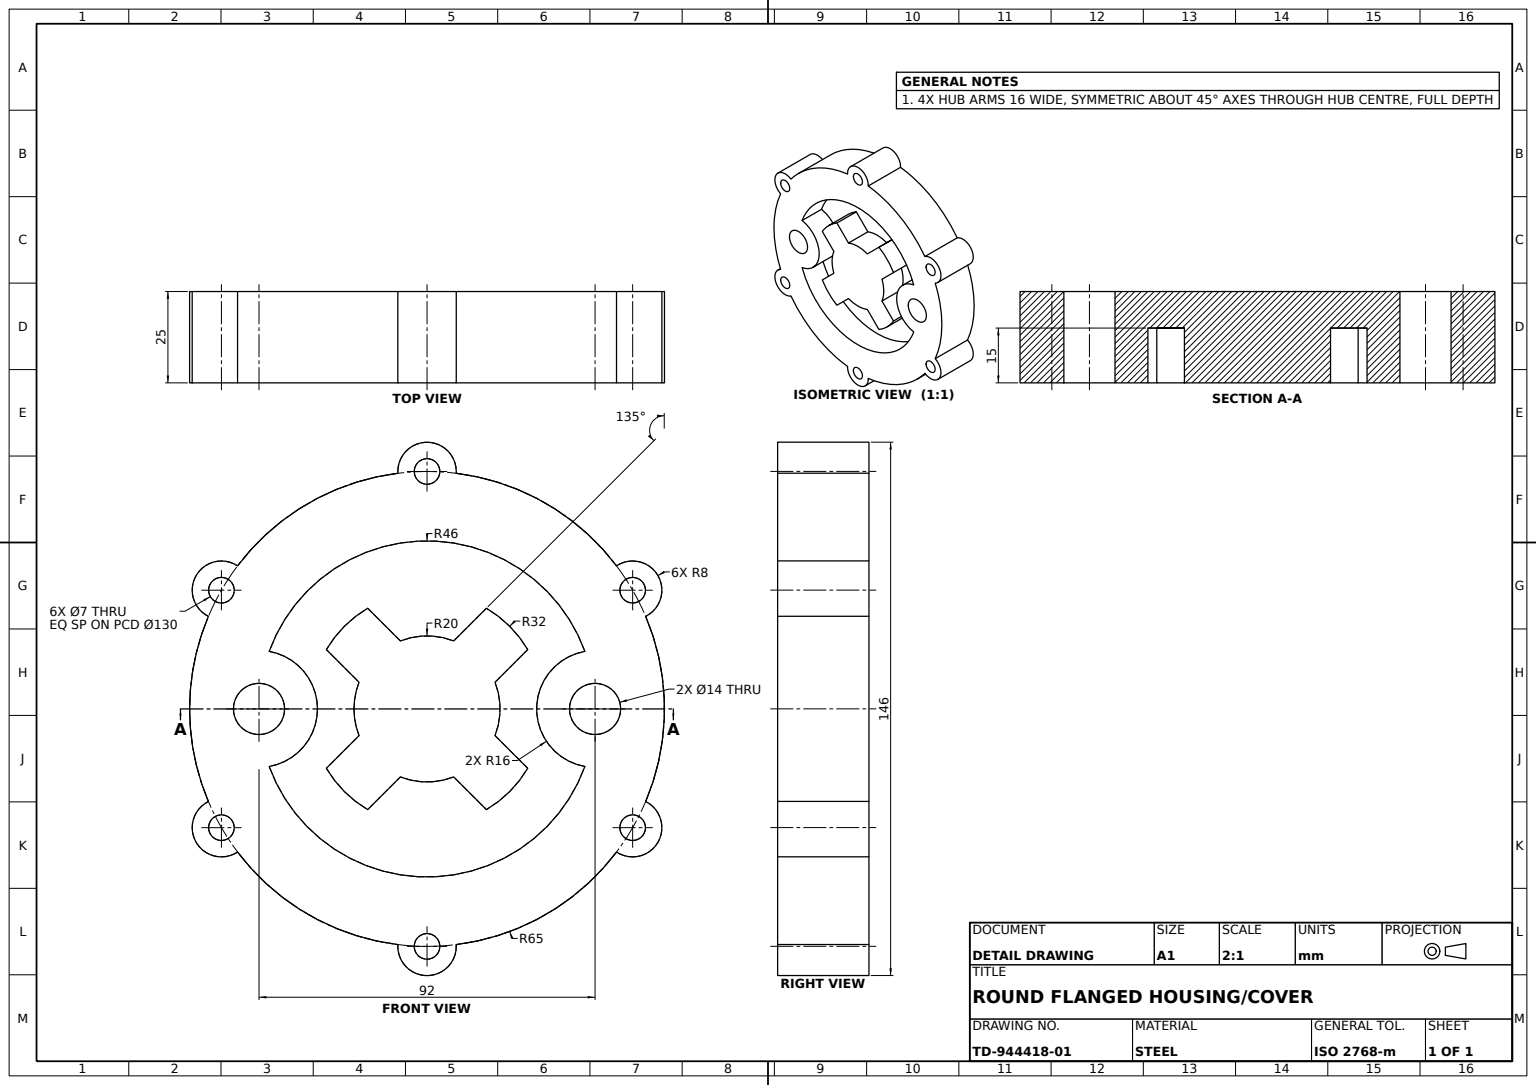
solid
v1 (52.791651,-32.5,25)
v2 (52.791651,-32.5,0)
e1 v1 v2 LINE
v3 (59.791651,-32.5,0)
e2 v3 v2 CIRCLE(AX(P(56.291651,-32.5,0),D(0,0,1),D(1,0,0)),3.5)
v4 (59.791651,-32.5,25)
e3 v4 v3 LINE
e4 v4 v1 CIRCLE(AX(P(56.291651,-32.5,25),D(0,0,1),D(1,0,0)),3.5)
face CYL(AX(P(56.291651,-32.5,25),D(0,0,-1),D(-1,0,0)),3.5) rev [e1 -e2 -e3 e4]
v5 (-16.252048,27.565757,25)
v6 (-16.252048,27.565757,10)
e5 v5 v6 LINE
v7 (-27.565757,16.252048,10)
e6 v6 v7 CIRCLE(AX(P(0,0,10),D(0,0,1),D(1,0,0)),32)
v8 (-27.565757,16.252048,25)
e7 v8 v7 LINE
e8 v5 v8 CIRCLE(AX(P(0,0,25),D(0,0,1),D(1,0,0)),32)
face CYL(AX(P(0,0,25),D(0,0,-1),D(-1,0,0)),32) [e5 e6 -e7 -e8]
v9 (-30,0,10)
v10 (-43.217391,-15.756176,10)
e9 v9 v10 CIRCLE(AX(P(-46,0,10),D(0,0,-1),D(-1,0,0)),16)
v11 (-30,0,25)
e10 v9 v11 LINE
v12 (-43.217391,-15.756176,25)
e11 v11 v12 CIRCLE(AX(P(-46,0,25),D(0,0,-1),D(-1,0,0)),16)
e12 v10 v12 LINE
face CYL(AX(P(-46,0,10),D(0,0,1),D(1,0,0)),16) [-e9 e10 e11 -e12]
v13 (-3.5,-65,25)
v14 (-3.5,-65,0)
e13 v13 v14 LINE
v15 (3.5,-65,25)
e14 v13 v15 CIRCLE(AX(P(0,-65,25),D(0,0,1),D(1,0,0)),3.5)
v16 (3.5,-65,0)
e15 v15 v16 LINE
e16 v14 v16 CIRCLE(AX(P(0,-65,0),D(0,0,1),D(1,0,0)),3.5)
face CYL(AX(P(0,-65,25),D(0,0,-1),D(-1,0,0)),3.5) rev [-e13 e14 e15 -e16]
v17 (-52.791651,32.5,25)
v18 (-52.791651,32.5,0)
e17 v17 v18 LINE
v19 (-59.791651,32.5,0)
e18 v19 v18 CIRCLE(AX(P(-56.291651,32.5,0),D(0,0,1),D(1,0,0)),3.5)
v20 (-59.791651,32.5,25)
e19 v20 v19 LINE
e20 v20 v17 CIRCLE(AX(P(-56.291651,32.5,25),D(0,0,1),D(1,0,0)),3.5)
face CYL(AX(P(-56.291651,32.5,25),D(0,0,-1),D(-1,0,0)),3.5) rev [e17 -e18 -e19 e20]
v21 (8,65,0)
v22 (-8,65,0)
e21 v21 v22 CIRCLE(AX(P(0,65,0),D(0,0,1),D(1,0,0)),8)
v23 (-8,65,25)
e22 v23 v22 LINE
v24 (8,65,25)
e23 v24 v23 CIRCLE(AX(P(0,65,25),D(0,0,1),D(1,0,0)),8)
e24 v24 v21 LINE
face CYL(AX(P(0,65,25),D(0,0,-1),D(-1,0,0)),8) [e21 -e22 -e23 e24]
v25 (7.304627,-18.618336,25)
v26 (7.304627,-18.618336,10)
e25 v25 v26 LINE
v27 (-7.304627,-18.618336,25)
e26 v27 v25 CIRCLE(AX(P(0,0,25),D(0,0,1),D(1,0,0)),20)
v28 (-7.304627,-18.618336,10)
e27 v27 v28 LINE
e28 v28 v26 CIRCLE(AX(P(0,0,10),D(0,0,1),D(1,0,0)),20)
face CYL(AX(P(0,0,25),D(0,0,-1),D(-1,0,0)),20) [-e25 -e26 e27 e28]
v29 (-53,0,0)
v30 (-53,0,25)
e29 v29 v30 LINE
v31 (-39,0,25)
e30 v30 v31 CIRCLE(AX(P(-46,0,25),D(0,0,1),D(-1,0,0)),7)
v32 (-39,0,0)
e31 v32 v31 LINE
e32 v29 v32 CIRCLE(AX(P(-46,0,0),D(0,0,1),D(-1,0,0)),7)
face CYL(AX(P(-46,0,0),D(0,0,1),D(1,0,0)),7) rev [e29 e30 -e31 -e32]
v33 (-59.857719,-25.338774,25)
v34 (-64.291651,-32.5,25)
e33 v33 v34 CIRCLE(AX(P(-56.291651,-32.5,25),D(0,0,1),D(1,0,0)),8)
v35 (-59.857719,-25.338774,0)
e34 v33 v35 LINE
v36 (-64.291651,-32.5,0)
e35 v35 v36 CIRCLE(AX(P(-56.291651,-32.5,0),D(0,0,1),D(1,0,0)),8)
e36 v34 v36 LINE
face CYL(AX(P(-56.291651,-32.5,25),D(0,0,-1),D(-1,0,0)),8) [-e33 e34 e35 -e36]
v37 (59.857719,-25.338774,25)
v38 (59.857719,-25.338774,0)
e37 v37 v38 LINE
v39 (59.857719,25.338774,0)
e38 v38 v39 CIRCLE(AX(P(0,0,0),D(0,0,1),D(1,0,0)),65)
v40 (59.857719,25.338774,25)
e39 v40 v39 LINE
e40 v37 v40 CIRCLE(AX(P(0,0,25),D(0,0,1),D(1,0,0)),65)
face CYL(AX(P(0,0,25),D(0,0,-1),D(-1,0,0)),65) [e37 e38 -e39 -e40]
v41 (7.984838,64.507692,0)
e41 v41 v21 CIRCLE(AX(P(0,65,0),D(0,0,1),D(1,0,0)),8)
v42 (7.984838,64.507692,25)
e42 v42 v24 CIRCLE(AX(P(0,65,25),D(0,0,1),D(1,0,0)),8)
e43 v42 v41 LINE
face CYL(AX(P(0,65,25),D(0,0,-1),D(-1,0,0)),8) [e41 -e24 -e42 e43]
v43 (-51.872881,-39.168918,0)
e44 v36 v43 CIRCLE(AX(P(-56.291651,-32.5,0),D(0,0,1),D(1,0,0)),8)
v44 (-51.872881,-39.168918,25)
e45 v44 v43 LINE
e46 v34 v44 CIRCLE(AX(P(-56.291651,-32.5,25),D(0,0,1),D(1,0,0)),8)
face CYL(AX(P(-56.291651,-32.5,25),D(0,0,-1),D(-1,0,0)),8) [e36 e44 -e45 -e46]
v45 (7.304627,18.618336,25)
v46 (7.304627,18.618336,10)
e47 v45 v46 LINE
v47 (-7.304627,18.618336,10)
e48 v46 v47 CIRCLE(AX(P(0,0,10),D(0,0,1),D(1,0,0)),20)
v48 (-7.304627,18.618336,25)
e49 v48 v47 LINE
e50 v45 v48 CIRCLE(AX(P(0,0,25),D(0,0,1),D(1,0,0)),20)
face CYL(AX(P(0,0,25),D(0,0,-1),D(-1,0,0)),20) [e47 e48 -e49 -e50]
v49 (39,0,0)
v50 (39,0,25)
e51 v49 v50 LINE
v51 (53,0,0)
e52 v51 v49 CIRCLE(AX(P(46,0,0),D(0,0,1),D(1,0,0)),7)
v52 (53,0,25)
e53 v51 v52 LINE
e54 v52 v50 CIRCLE(AX(P(46,0,25),D(0,0,1),D(1,0,0)),7)
face CYL(AX(P(46,0,0),D(0,0,1),D(1,0,0)),7) rev [-e51 -e52 e53 e54]
v53 (-3.5,65,25)
v54 (3.5,65,25)
e55 v53 v54 CIRCLE(AX(P(0,65,25),D(0,0,1),D(1,0,0)),3.5)
e56 v54 v53 CIRCLE(AX(P(0,65,25),D(0,0,1),D(1,0,0)),3.5)
v55 (-52.791651,-32.5,25)
v56 (-59.791651,-32.5,25)
e57 v55 v56 CIRCLE(AX(P(-56.291651,-32.5,25),D(0,0,1),D(1,0,0)),3.5)
e58 v56 v55 CIRCLE(AX(P(-56.291651,-32.5,25),D(0,0,1),D(1,0,0)),3.5)
e59 v15 v13 CIRCLE(AX(P(0,-65,25),D(0,0,1),D(1,0,0)),3.5)
e60 v17 v20 CIRCLE(AX(P(-56.291651,32.5,25),D(0,0,1),D(1,0,0)),3.5)
e61 v31 v30 CIRCLE(AX(P(-46,0,25),D(0,0,1),D(-1,0,0)),7)
v57 (59.791651,32.5,25)
v58 (52.791651,32.5,25)
e62 v57 v58 CIRCLE(AX(P(56.291651,32.5,25),D(0,0,1),D(1,0,0)),3.5)
e63 v58 v57 CIRCLE(AX(P(56.291651,32.5,25),D(0,0,1),D(1,0,0)),3.5)
e64 v50 v52 CIRCLE(AX(P(46,0,25),D(0,0,1),D(1,0,0)),7)
v59 (-43.217391,15.756176,25)
e65 v59 v11 CIRCLE(AX(P(-46,0,25),D(0,0,-1),D(-1,0,0)),16)
v60 (43.217391,15.756176,25)
e66 v60 v59 CIRCLE(AX(P(0,0,25),D(0,0,1),D(1,0,0)),46)
v61 (43.217391,-15.756176,25)
e67 v61 v60 CIRCLE(AX(P(46,0,25),D(0,0,-1),D(1,0,0)),16)
e68 v12 v61 CIRCLE(AX(P(0,0,25),D(0,0,1),D(1,0,0)),46)
v62 (51.872881,39.168918,25)
e69 v62 v42 CIRCLE(AX(P(0,0,25),D(0,0,1),D(1,0,0)),65)
v63 (-7.984838,64.507692,25)
e70 v23 v63 CIRCLE(AX(P(0,65,25),D(0,0,1),D(1,0,0)),8)
v64 (-51.872881,39.168918,25)
e71 v63 v64 CIRCLE(AX(P(0,0,25),D(0,0,1),D(1,0,0)),65)
v65 (-64.291651,32.5,25)
e72 v64 v65 CIRCLE(AX(P(-56.291651,32.5,25),D(0,0,1),D(1,0,0)),8)
v66 (-59.857719,25.338774,25)
e73 v65 v66 CIRCLE(AX(P(-56.291651,32.5,25),D(0,0,1),D(1,0,0)),8)
v67 (-65,0,25)
e74 v66 v67 CIRCLE(AX(P(0,0,25),D(0,0,1),D(1,0,0)),65)
e75 v67 v33 CIRCLE(AX(P(0,0,25),D(0,0,1),D(1,0,0)),65)
v68 (-7.984838,-64.507692,25)
e76 v44 v68 CIRCLE(AX(P(0,0,25),D(0,0,1),D(1,0,0)),65)
v69 (-8,-65,25)
e77 v68 v69 CIRCLE(AX(P(0,-65,25),D(0,0,1),D(1,0,0)),8)
v70 (8,-65,25)
e78 v69 v70 CIRCLE(AX(P(0,-65,25),D(0,0,1),D(1,0,0)),8)
v71 (7.984838,-64.507692,25)
e79 v70 v71 CIRCLE(AX(P(0,-65,25),D(0,0,1),D(1,0,0)),8)
v72 (51.872881,-39.168918,25)
e80 v71 v72 CIRCLE(AX(P(0,0,25),D(0,0,1),D(1,0,0)),65)
e81 v72 v37 CIRCLE(AX(P(56.291651,-32.5,25),D(0,0,1),D(1,0,0)),8)
e82 v40 v62 CIRCLE(AX(P(56.291651,32.5,25),D(0,0,1),D(1,0,0)),8)
e83 v1 v4 CIRCLE(AX(P(56.291651,-32.5,25),D(0,0,1),D(1,0,0)),3.5)
face PLANE(AX(P(28.145826,-16.25,25),D(0,0,1),D(1,0,0))) [-e55 -e56] [-e57 -e58] [-e14 -e59] [-e20 -e60] [-e30 -e61] [-e62 -e63] [-e64 -e54] [-e65 -e66 -e67 -e68 -e11] [e69 e42 e23 e70 e71 e72 e73 e74 e75 e33 e46 e76 e77 e78 e79 e80 e81 e40 e82] [-e83 -e4]
v73 (-8,-65,0)
e84 v69 v73 LINE
v74 (8,-65,0)
e85 v73 v74 CIRCLE(AX(P(0,-65,0),D(0,0,1),D(1,0,0)),8)
e86 v70 v74 LINE
face CYL(AX(P(0,-65,25),D(0,0,-1),D(-1,0,0)),8) [e84 e85 -e86 -e78]
v75 (18.618336,7.304627,25)
v76 (18.618336,7.304627,10)
e87 v75 v76 LINE
v77 (18.618336,-7.304627,25)
e88 v77 v75 CIRCLE(AX(P(0,0,25),D(0,0,1),D(1,0,0)),20)
v78 (18.618336,-7.304627,10)
e89 v77 v78 LINE
e90 v78 v76 CIRCLE(AX(P(0,0,10),D(0,0,1),D(1,0,0)),20)
face CYL(AX(P(0,0,25),D(0,0,-1),D(-1,0,0)),20) [-e87 -e88 e89 e90]
v79 (-27.565757,-16.252048,25)
v80 (-16.252048,-27.565757,25)
e91 v79 v80 CIRCLE(AX(P(0,0,25),D(0,0,1),D(1,0,0)),32)
v81 (-27.565757,-16.252048,10)
e92 v79 v81 LINE
v82 (-16.252048,-27.565757,10)
e93 v81 v82 CIRCLE(AX(P(0,0,10),D(0,0,1),D(1,0,0)),32)
e94 v80 v82 LINE
face CYL(AX(P(0,0,25),D(0,0,-1),D(-1,0,0)),32) [-e91 e92 e93 -e94]
v83 (16.252048,27.565757,25)
v84 (16.252048,27.565757,10)
e95 v83 v84 LINE
e96 v84 v46 LINE
e97 v83 v45 LINE
face PLANE(AX(P(7.304627,18.618336,25),D(0.707106781,-0.707106781,0),D(0.707106781,0.707106781,0))) rev [e95 e96 -e47 -e97]
e98 v80 v27 LINE
e99 v82 v28 LINE
face PLANE(AX(P(-7.304627,-18.618336,25),D(-0.707106781,0.707106781,0),D(-0.707106781,-0.707106781,0))) rev [-e27 -e98 e94 e99]
v85 (51.872881,39.168918,0)
e100 v39 v85 CIRCLE(AX(P(56.291651,32.5,0),D(0,0,1),D(1,0,0)),8)
e101 v62 v85 LINE
face CYL(AX(P(56.291651,32.5,25),D(0,0,-1),D(-1,0,0)),8) [-e82 e39 e100 -e101]
v86 (51.872881,-39.168918,0)
e102 v72 v86 LINE
e103 v86 v38 CIRCLE(AX(P(56.291651,-32.5,0),D(0,0,1),D(1,0,0)),8)
face CYL(AX(P(56.291651,-32.5,25),D(0,0,-1),D(-1,0,0)),8) [e102 e103 -e37 -e81]
v87 (-64.291651,32.5,0)
v88 (-59.857719,25.338774,0)
e104 v87 v88 CIRCLE(AX(P(-56.291651,32.5,0),D(0,0,1),D(1,0,0)),8)
e105 v66 v88 LINE
e106 v65 v87 LINE
face CYL(AX(P(-56.291651,32.5,25),D(0,0,-1),D(-1,0,0)),8) [e104 -e105 -e73 e106]
e107 v85 v41 CIRCLE(AX(P(0,0,0),D(0,0,1),D(1,0,0)),65)
face CYL(AX(P(0,0,25),D(0,0,-1),D(-1,0,0)),65) [e107 -e43 -e69 e101]
v89 (27.565757,16.252048,25)
e108 v75 v89 LINE
e109 v89 v83 CIRCLE(AX(P(0,0,25),D(0,0,1),D(1,0,0)),32)
e110 v48 v5 LINE
v90 (-18.618336,7.304627,25)
e111 v8 v90 LINE
v91 (-20,0,25)
e112 v90 v91 CIRCLE(AX(P(0,0,25),D(0,0,1),D(1,0,0)),20)
v92 (-18.618336,-7.304627,25)
e113 v91 v92 CIRCLE(AX(P(0,0,25),D(0,0,1),D(1,0,0)),20)
e114 v92 v79 LINE
v93 (16.252048,-27.565757,25)
e115 v25 v93 LINE
v94 (27.565757,-16.252048,25)
e116 v93 v94 CIRCLE(AX(P(0,0,25),D(0,0,1),D(1,0,0)),32)
e117 v94 v77 LINE
face PLANE(AX(P(0,0,25),D(0,0,1),D(1,0,0))) [e88 e108 e109 e97 e50 e110 e8 e111 e112 e113 e114 e91 e98 e26 e115 e116 e117]
v95 (-20,0,10)
e118 v91 v95 LINE
v96 (-18.618336,-7.304627,10)
e119 v95 v96 CIRCLE(AX(P(0,0,10),D(0,0,1),D(1,0,0)),20)
e120 v92 v96 LINE
face CYL(AX(P(0,0,25),D(0,0,-1),D(-1,0,0)),20) [e118 e119 -e120 -e113]
v97 (-59.791651,-32.5,0)
e121 v56 v97 LINE
v98 (-52.791651,-32.5,0)
e122 v98 v97 CIRCLE(AX(P(-56.291651,-32.5,0),D(0,0,1),D(1,0,0)),3.5)
e123 v55 v98 LINE
face CYL(AX(P(-56.291651,-32.5,25),D(0,0,-1),D(-1,0,0)),3.5) rev [e121 -e122 -e123 e57]
e124 v32 v29 CIRCLE(AX(P(-46,0,0),D(0,0,1),D(-1,0,0)),7)
face CYL(AX(P(-46,0,0),D(0,0,1),D(1,0,0)),7) rev [-e29 -e124 e31 e61]
v99 (3.5,65,0)
e125 v54 v99 LINE
v100 (-3.5,65,0)
e126 v100 v99 CIRCLE(AX(P(0,65,0),D(0,0,1),D(1,0,0)),3.5)
e127 v53 v100 LINE
face CYL(AX(P(0,65,25),D(0,0,-1),D(-1,0,0)),3.5) rev [e55 e125 -e126 -e127]
v101 (-7.984838,-64.507692,0)
e128 v43 v101 CIRCLE(AX(P(0,0,0),D(0,0,1),D(1,0,0)),65)
e129 v68 v101 LINE
face CYL(AX(P(0,0,25),D(0,0,-1),D(-1,0,0)),65) [e45 e128 -e129 -e76]
v102 (52.791651,32.5,0)
v103 (59.791651,32.5,0)
e130 v102 v103 CIRCLE(AX(P(56.291651,32.5,0),D(0,0,1),D(1,0,0)),3.5)
e131 v58 v102 LINE
e132 v57 v103 LINE
face CYL(AX(P(56.291651,32.5,25),D(0,0,-1),D(-1,0,0)),3.5) rev [-e130 -e131 e63 e132]
v104 (43.217391,15.756176,10)
v105 (-43.217391,15.756176,10)
e133 v104 v105 CIRCLE(AX(P(0,0,10),D(0,0,1),D(1,0,0)),46)
e134 v104 v60 LINE
e135 v105 v59 LINE
face CYL(AX(P(0,0,10),D(0,0,1),D(1,0,0)),46) rev [-e133 e134 e66 -e135]
v106 (-65,0,0)
e136 v67 v106 LINE
e137 v106 v35 CIRCLE(AX(P(0,0,0),D(0,0,1),D(1,0,0)),65)
face CYL(AX(P(0,0,25),D(0,0,-1),D(-1,0,0)),65) [e136 e137 -e34 -e75]
e138 v105 v9 CIRCLE(AX(P(-46,0,10),D(0,0,-1),D(-1,0,0)),16)
face CYL(AX(P(-46,0,10),D(0,0,1),D(1,0,0)),16) [e65 -e10 -e138 e135]
v107 (16.252048,-27.565757,10)
e139 v26 v107 LINE
e140 v93 v107 LINE
face PLANE(AX(P(7.304627,-18.618336,25),D(0.707106781,0.707106781,0),D(-0.707106781,0.707106781,0))) rev [e25 e139 -e140 -e115]
v108 (-51.872881,39.168918,0)
e141 v64 v108 LINE
e142 v108 v87 CIRCLE(AX(P(-56.291651,32.5,0),D(0,0,1),D(1,0,0)),8)
face CYL(AX(P(-56.291651,32.5,25),D(0,0,-1),D(-1,0,0)),8) [-e106 -e72 e141 e142]
v109 (27.565757,-16.252048,10)
e143 v109 v78 LINE
e144 v94 v109 LINE
face PLANE(AX(P(18.618336,-7.304627,25),D(-0.707106781,-0.707106781,0),D(0.707106781,-0.707106781,0))) rev [e143 -e89 -e117 e144]
v110 (-7.984838,64.507692,0)
e145 v22 v110 CIRCLE(AX(P(0,65,0),D(0,0,1),D(1,0,0)),8)
e146 v63 v110 LINE
face CYL(AX(P(0,65,25),D(0,0,-1),D(-1,0,0)),8) [e145 -e146 -e70 e22]
e147 v16 v14 CIRCLE(AX(P(0,-65,0),D(0,0,1),D(1,0,0)),3.5)
face CYL(AX(P(0,-65,25),D(0,0,-1),D(-1,0,0)),3.5) rev [e59 e13 -e147 -e15]
e148 v47 v6 LINE
face PLANE(AX(P(-7.304627,18.618336,25),D(-0.707106781,-0.707106781,0),D(0.707106781,-0.707106781,0))) rev [-e5 -e110 e49 e148]
v111 (7.984838,-64.507692,0)
e149 v74 v111 CIRCLE(AX(P(0,-65,0),D(0,0,1),D(1,0,0)),8)
e150 v71 v111 LINE
face CYL(AX(P(0,-65,25),D(0,0,-1),D(-1,0,0)),8) [-e79 e86 e149 -e150]
e151 v107 v109 CIRCLE(AX(P(0,0,10),D(0,0,1),D(1,0,0)),32)
face CYL(AX(P(0,0,25),D(0,0,-1),D(-1,0,0)),32) [-e144 -e116 e140 e151]
e152 v88 v106 CIRCLE(AX(P(0,0,0),D(0,0,1),D(1,0,0)),65)
face CYL(AX(P(0,0,25),D(0,0,-1),D(-1,0,0)),65) [-e74 e105 e152 -e136]
v112 (-18.618336,7.304627,10)
e153 v90 v112 LINE
e154 v112 v95 CIRCLE(AX(P(0,0,10),D(0,0,1),D(1,0,0)),20)
face CYL(AX(P(0,0,25),D(0,0,-1),D(-1,0,0)),20) [e153 e154 -e118 -e112]
e155 v2 v3 CIRCLE(AX(P(56.291651,-32.5,0),D(0,0,1),D(1,0,0)),3.5)
face CYL(AX(P(56.291651,-32.5,25),D(0,0,-1),D(-1,0,0)),3.5) rev [-e1 e83 e3 -e155]
v113 (27.565757,16.252048,10)
e156 v89 v113 LINE
e157 v113 v84 CIRCLE(AX(P(0,0,10),D(0,0,1),D(1,0,0)),32)
face CYL(AX(P(0,0,25),D(0,0,-1),D(-1,0,0)),32) [-e95 -e109 e156 e157]
e158 v103 v102 CIRCLE(AX(P(56.291651,32.5,0),D(0,0,1),D(1,0,0)),3.5)
e159 v18 v19 CIRCLE(AX(P(-56.291651,32.5,0),D(0,0,1),D(1,0,0)),3.5)
e160 v99 v100 CIRCLE(AX(P(0,65,0),D(0,0,1),D(1,0,0)),3.5)
e161 v97 v98 CIRCLE(AX(P(-56.291651,-32.5,0),D(0,0,1),D(1,0,0)),3.5)
e162 v49 v51 CIRCLE(AX(P(46,0,0),D(0,0,1),D(1,0,0)),7)
e163 v110 v108 CIRCLE(AX(P(0,0,0),D(0,0,1),D(1,0,0)),65)
e164 v111 v86 CIRCLE(AX(P(0,0,0),D(0,0,1),D(1,0,0)),65)
e165 v101 v73 CIRCLE(AX(P(0,-65,0),D(0,0,1),D(1,0,0)),8)
face PLANE(AX(P(28.145826,-16.25,0),D(0,0,1),D(1,0,0))) rev [e158 e130] [e2 e155] [e159 e18] [e160 e126] [e16 e147] [e161 e122] [e162 e52] [-e35 -e137 -e152 -e104 -e142 -e163 -e145 -e21 -e41 -e107 -e100 -e38 -e103 -e164 -e149 -e85 -e165 -e128 -e44] [e32 e124]
face CYL(AX(P(56.291651,32.5,25),D(0,0,-1),D(-1,0,0)),3.5) rev [e131 -e158 -e132 e62]
v114 (43.217391,-15.756176,10)
e166 v10 v114 CIRCLE(AX(P(0,0,10),D(0,0,1),D(1,0,0)),46)
e167 v114 v61 LINE
face CYL(AX(P(0,0,10),D(0,0,1),D(1,0,0)),46) rev [-e166 e12 e68 -e167]
face CYL(AX(P(-56.291651,32.5,25),D(0,0,-1),D(-1,0,0)),3.5) rev [-e17 e60 e19 -e159]
face CYL(AX(P(0,-65,25),D(0,0,-1),D(-1,0,0)),8) [e165 -e84 -e77 e129]
face CYL(AX(P(46,0,0),D(0,0,1),D(1,0,0)),7) rev [e64 -e53 -e162 e51]
e168 v7 v112 LINE
face PLANE(AX(P(-18.618336,7.304627,25),D(0.707106781,0.707106781,0),D(-0.707106781,0.707106781,0))) rev [e7 e168 -e153 -e111]
face CYL(AX(P(0,65,25),D(0,0,-1),D(-1,0,0)),3.5) rev [-e160 -e125 e56 e127]
e169 v114 v104 CIRCLE(AX(P(46,0,10),D(0,0,-1),D(1,0,0)),16)
face CYL(AX(P(46,0,10),D(0,0,1),D(1,0,0)),16) [e167 e67 -e134 -e169]
e170 v76 v113 LINE
face PLANE(AX(P(18.618336,7.304627,25),D(-0.707106781,0.707106781,0),D(-0.707106781,-0.707106781,0))) rev [e87 e170 -e156 -e108]
e171 v96 v81 LINE
face PLANE(AX(P(23,0,10),D(0,0,1),D(1,0,0))) [-e171 -e119 -e154 -e168 -e6 -e148 -e48 -e96 -e157 -e170 -e90 -e143 -e151 -e139 -e28 -e99 -e93] [e133 e138 e9 e166 e169]
face CYL(AX(P(0,0,25),D(0,0,-1),D(-1,0,0)),65) [e150 e164 -e102 -e80]
face CYL(AX(P(-56.291651,-32.5,25),D(0,0,-1),D(-1,0,0)),3.5) rev [-e121 e58 e123 -e161]
face PLANE(AX(P(-18.618336,-7.304627,25),D(0.707106781,-0.707106781,0),D(0.707106781,0.707106781,0))) rev [e171 -e92 -e114 e120]
face CYL(AX(P(0,0,25),D(0,0,-1),D(-1,0,0)),65) [e163 -e141 -e71 e146]
